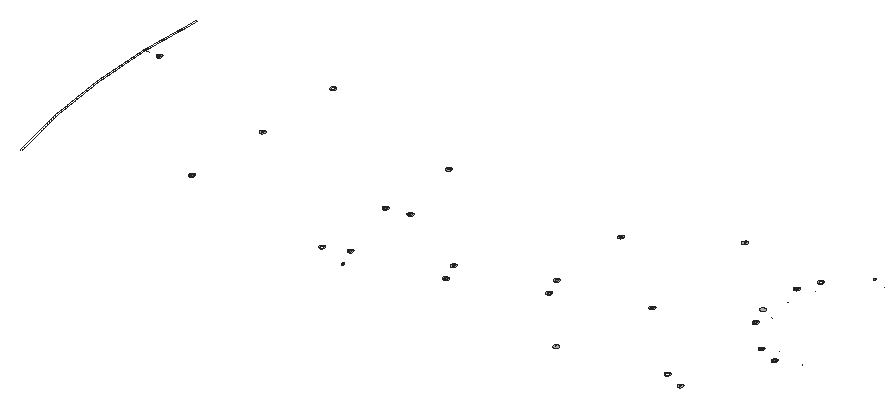
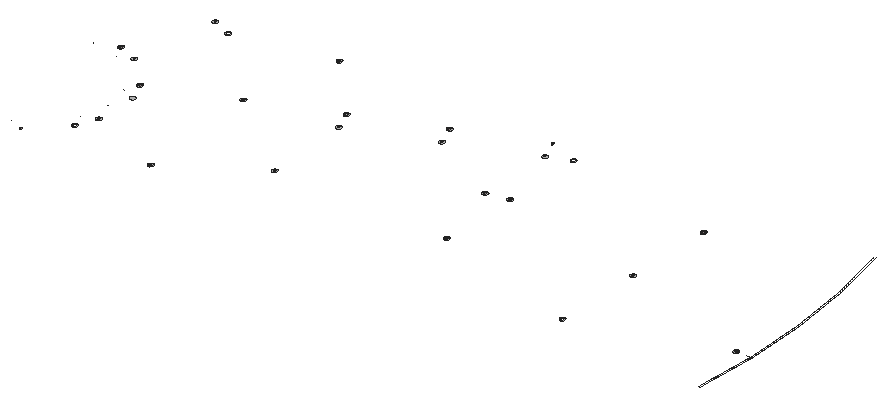
# SketchUp Ruby script. Lengths in inches.
U = 1.inch
M = Sketchup.active_model
def pt(a) = Geom::Point3d.new(a.map { |v| v * U })
def face(e, loops, mat)
  f = e.add_face(loops[0].map { |a| pt(a) })
  loops[1..].each { |l| e.add_face(l.map { |a| pt(a) }).erase! }
  f.material = f.back_material = mat if mat
  f
end
# faces: each face lists its corners as indices into pts; further lists are holes
def faces(e, pts, list, mat = nil) = list.each { |f| face(e, (f[0].is_a?(Array) ? f : [f]).map { |l| l.map { |i| pts[i] } }, mat) }
# xy, xz, yz: faces in a plane at the given z, y or x. An outline is a flat list of corners, or four numbers for a rectangle; further outlines are holes
def ring(l) = l.size == 4 ? [[l[0], l[1]], [l[2], l[1]], [l[2], l[3]], [l[0], l[3]]] : l.each_slice(2).to_a
def flat(e, list, mat, &to3) = list.each { |f| face(e, (f[0].is_a?(Array) ? f : [f]).map { |l| ring(l).map { |u, v| to3.(u, v) } }, mat) }
def xy(e, z, list, mat = nil) = flat(e, list, mat) { |x, y| [x, y, z] }
def xz(e, y, list, mat = nil) = flat(e, list, mat) { |x, z| [x, y, z] }
def yz(e, x, list, mat = nil) = flat(e, list, mat) { |y, z| [x, y, z] }
def lines(e, pts, list) = list.each { |a, b| e.add_line(pt(pts[a]), pt(pts[b])) }
# prism: a flat outline (further loops are holes) pulled along v
def prism(e, loops, v, mat = nil)
  f = face(e, loops, mat); d = Geom::Vector3d.new(v.map { |x| x * U })
  f.pushpull(f.normal.samedirection?(d) ? d.length : -d.length)
end
def box(e, o, s, mat = nil) = prism(e, [[o, [o[0] + s[0], o[1], o[2]], [o[0] + s[0], o[1] + s[1], o[2]], [o[0], o[1] + s[1], o[2]]]], [0, 0, s[2]], mat)
def at(x, y, z, deg = 0) = Geom::Transformation.translation(pt([x, y, z])) * Geom::Transformation.rotation(ORIGIN, Z_AXIS, deg.degrees)
def axes(o, x, y, z) = Geom::Transformation.new([*x, 0, *y, 0, *z, 0, *pt(o).to_a, 1])
def part(name) = M.definitions.add(name)
# library, detail: a bought-in or finely detailed component or shape, given as its bounding box
def library(name, o, s) = part(name).tap { |d| box(d.entities, o, s) }
def detail(e, o, s) = box(e.add_group.entities, o, s)
def put(e, d, t, mat = nil) = e.add_instance(d, t).tap { |i| i.material = mat if mat }
def group(e, t, mat = nil) = e.add_group.tap { |g| g.transformation = t; g.material = mat if mat }.entities
root = M.entities
M.materials.add("[Asphalt_Stamped_Brick]").color = [149, 133, 134]
M.materials.add("[Metal_Steel_Textured_White]").color = [191, 191, 191]
xy(root,3.625,[[147.823,157.497,147.818,157.498,147.8125,157.5,147.809,157.503,147.805,157.507,147.803,157.512,147.803,157.522,147.805,157.527,147.809,157.531,147.8125,157.535,147.818,157.537,147.828,157.537,147.833,157.535,147.837,157.531,147.84,157.527,147.842,157.522,147.843,157.517,147.842,157.512,147.84,157.507,147.837,157.503,147.833,157.5,147.828,157.498],[135.246,157.754,135.241,157.755,135.236,157.757,135.232,157.76,135.229,157.764,135.227,157.769,135.226,157.774,135.227,157.779,135.229,157.784,135.232,157.788,135.236,157.791,135.241,157.793,135.246,157.794,135.252,157.793,135.256,157.791,135.261,157.788,135.264,157.784,135.266,157.779,135.266,157.769,135.264,157.764,135.261,157.76,135.256,157.757,135.252,157.755],[138.456,158.219,138.451,158.22,138.446,158.222,138.442,158.225,138.438,158.229,138.436,158.234,138.436,158.244,138.438,158.249,138.442,158.253,138.446,158.256,138.451,158.258,138.456,158.259,138.461,158.258,138.466,158.256,138.47,158.253,138.473,158.249,138.475,158.244,138.476,158.239,138.475,158.234,138.473,158.229,138.47,158.225,138.466,158.222,138.461,158.22],[128.792,158.391,128.787,158.392,128.782,158.394,128.778,158.397,128.775,158.401,128.773,158.406,128.772,158.411,128.773,158.416,128.775,158.421,128.778,158.425,128.782,158.429,128.787,158.431,128.798,158.431,128.802,158.429,128.807,158.425,128.81,158.421,128.812,158.416,128.8125,158.411,128.812,158.406,128.81,158.401,128.807,158.397,128.802,158.394,128.798,158.392],[138.145,158.957,138.14,158.959,138.136,158.963,138.133,158.967,138.131,158.971,138.13,158.977,138.131,158.982,138.133,158.987,138.136,158.991,138.14,158.994,138.145,158.996,138.15,158.997,138.155,158.996,138.16,158.994,138.164,158.991,138.168,158.987,138.17,158.977,138.169,158.971,138.168,158.967,138.16,158.959,138.155,158.957],
  [141.054,160.159,141.049,160.16,141.044,160.162,141.04,160.165,141.037,160.169,141.035,160.174,141.034,160.179,141.035,160.185,141.037,160.189,141.04,160.194,141.044,160.197,141.049,160.199,141.059,160.199,141.064,160.197,141.068,160.194,141.071,160.189,141.073,160.185,141.074,160.179,141.073,160.174,141.071,160.169,141.068,160.165,141.064,160.162,141.059,160.16],[134.448,160.39,134.443,160.391,134.438,160.393,134.434,160.396,134.431,160.4,134.429,160.405,134.428,160.41,134.429,160.415,134.431,160.42,134.434,160.424,134.438,160.428,134.443,160.43,134.453,160.43,134.458,160.428,134.462,160.424,134.465,160.42,134.467,160.415,134.468,160.41,134.467,160.405,134.465,160.4,134.462,160.396,134.458,160.393,134.453,160.391],[149.025,160.401,149.02,160.402,149.015,160.404,149.011,160.407,149.008,160.411,149.006,160.416,149.005,160.421,149.006,160.426,149.008,160.431,149.011,160.435,149.015,160.438,149.02,160.44,149.025,160.441,149.031,160.44,149.035,160.438,149.04,160.435,149.043,160.431,149.045,160.426,149.045,160.416,149.043,160.411,149.04,160.407,149.035,160.404,149.031,160.402],[135.241,160.556,135.236,160.558,135.232,160.562,135.229,160.566,135.227,160.57,135.226,160.576,135.227,160.581,135.229,160.586,135.232,160.59,135.236,160.593,135.241,160.595,135.246,160.596,135.252,160.595,135.256,160.593,135.261,160.59,135.264,160.586,135.266,160.581,135.266,160.57,135.264,160.566,135.261,160.562,135.256,160.558,135.252,160.556],[144.258,160.625,144.253,160.627,144.249,160.63,144.246,160.635,144.244,160.639,144.243,160.645,144.244,160.65,144.246,160.655,144.249,160.659,144.253,160.662,144.258,160.664,144.263,160.665,144.269,160.664,144.273,160.662,144.277,160.659,144.281,160.655,144.283,160.65,144.283,160.639,144.281,160.635,144.277,160.63,144.273,160.627,144.269,160.625],
  [148.283,160.707,148.278,160.709,148.274,160.713,148.271,160.717,148.269,160.721,148.268,160.727,148.269,160.732,148.271,160.737,148.274,160.741,148.278,160.744,148.283,160.746,148.288,160.747,148.293,160.746,148.298,160.744,148.302,160.741,148.305,160.737,148.307,160.732,148.308,160.727,148.307,160.721,148.305,160.717,148.302,160.713,148.298,160.709,148.293,160.707],[128.792,161.702,128.787,161.703,128.782,161.705,128.778,161.708,128.775,161.712,128.773,161.717,128.772,161.722,128.773,161.727,128.775,161.732,128.778,161.736,128.782,161.739,128.787,161.741,128.792,161.742,128.798,161.741,128.802,161.739,128.807,161.736,128.81,161.732,128.812,161.727,128.8125,161.722,128.812,161.717,128.81,161.712,128.807,161.708,128.802,161.705,128.798,161.703],[147.167,161.827,147.162,161.828,147.157,161.83,147.153,161.833,147.15,161.837,147.148,161.842,147.147,161.847,147.148,161.852,147.15,161.857,147.153,161.861,147.157,161.865,147.162,161.867,147.172,161.867,147.177,161.865,147.181,161.861,147.184,161.857,147.186,161.852,147.187,161.847,147.186,161.842,147.184,161.837,147.181,161.833,147.177,161.83,147.172,161.828],[146.862,164.15,146.856,164.151,146.852,164.153,146.847,164.156,146.844,164.16,146.842,164.165,146.842,164.175,146.844,164.18,146.847,164.184,146.852,164.187,146.856,164.189,146.862,164.19,146.867,164.189,146.872,164.187,146.876,164.184,146.879,164.18,146.881,164.175,146.882,164.17,146.881,164.165,146.879,164.16,146.876,164.156,146.872,164.153,146.867,164.151],[143.953,165.353,143.948,165.355,143.944,165.359,143.941,165.363,143.939,165.367,143.938,165.373,143.939,165.378,143.941,165.383,143.944,165.387,143.948,165.39,143.953,165.392,143.958,165.393,143.963,165.392,143.968,165.39,143.972,165.387,143.975,165.383,143.977,165.378,143.978,165.373,143.977,165.367,143.975,165.363,143.972,165.359,143.968,165.355,143.963,165.353],
  [148.288,166.008,148.283,166.009,148.278,166.011,148.274,166.014,148.271,166.018,148.269,166.023,148.268,166.028,148.269,166.033,148.271,166.038,148.274,166.042,148.278,166.045,148.283,166.047,148.288,166.048,148.293,166.047,148.298,166.045,148.302,166.042,148.305,166.038,148.307,166.033,148.308,166.028,148.307,166.023,148.305,166.018,148.302,166.014,148.298,166.011,148.293,166.009]],"[Asphalt_Stamped_Brick]")
xy(root,3.625,[[[143.513,156.984,143.49,156.987,143.469,156.996,143.451,157.01,143.436,157.029,143.428,157.05,143.425,157.073,143.428,157.096,143.436,157.117,143.451,157.136,143.469,157.15,143.49,157.159,143.513,157.162,143.536,157.159,143.558,157.15,143.576,157.136,143.59,157.117,143.599,157.096,143.602,157.073,143.599,157.05,143.59,157.029,143.576,157.01,143.558,156.996,143.536,156.987],[143.513,156.985,143.536,156.988,143.557,156.997,143.576,157.011,143.59,157.029,143.598,157.05,143.601,157.073,143.598,157.096,143.59,157.117,143.576,157.135,143.557,157.149,143.536,157.158,143.513,157.161,143.491,157.158,143.469,157.149,143.451,157.135,143.437,157.117,143.428,157.096,143.425,157.073,143.428,157.05,143.437,157.029,143.451,157.011,143.469,156.997,143.491,156.988]],[[143.513,156.985,143.491,156.988,143.469,156.997,143.451,157.011,143.437,157.029,143.428,157.05,143.425,157.073,143.428,157.096,143.437,157.117,143.451,157.135,143.469,157.149,143.491,157.158,143.513,157.161,143.536,157.158,143.557,157.149,143.576,157.135,143.59,157.117,143.598,157.096,143.601,157.073,143.598,157.05,143.59,157.029,143.576,157.011,143.557,156.997,143.536,156.988],[143.513,157.036,143.523,157.038,143.532,157.041,143.539,157.047,143.545,157.055,143.549,157.063,143.55,157.073,143.549,157.082,143.545,157.091,143.539,157.099,143.532,157.105,143.523,157.108,143.513,157.11,143.504,157.108,143.495,157.105,143.488,157.099,143.482,157.091,143.478,157.082,143.477,157.073,143.478,157.063,143.482,157.055,143.488,157.047,143.495,157.041,143.504,157.038]],[[135.552,157,135.543,157.001,135.534,157.004,135.526,157.01,135.52,157.018,135.517,157.027,135.515,157.036,135.517,157.046,135.52,157.054,135.526,157.062,135.534,157.068,135.543,157.072,135.552,157.073,135.561,157.072,135.57,157.068,135.578,157.062,135.584,157.054,135.587,157.046,135.589,157.036,135.587,157.027,135.584,157.018,135.578,157.01,135.57,157.004,135.561,157.001],[135.552,157.016,135.557,157.017,135.562,157.019,135.566,157.022,135.569,157.026,135.571,157.031,135.572,157.036,135.571,157.041,135.569,157.046,135.566,157.05,135.562,157.053,135.557,157.055,135.552,157.056,135.547,157.055,135.542,157.053,135.538,157.05,135.535,157.046,135.533,157.041,135.532,157.036,135.533,157.031,135.535,157.026,135.538,157.022,135.542,157.019,135.547,157.017]],[135.552,157.016,135.547,157.017,135.542,157.019,135.538,157.022,135.535,157.026,135.533,157.031,135.532,157.036,135.533,157.041,135.535,157.046,135.538,157.05,135.542,157.053,135.547,157.055,135.552,157.056,135.557,157.055,135.562,157.053,135.566,157.05,135.569,157.046,135.571,157.041,135.572,157.036,135.571,157.031,135.569,157.026,135.566,157.022,135.562,157.019,135.557,157.017],[143.513,157.053,143.508,157.054,143.503,157.056,143.499,157.059,143.496,157.063,143.494,157.068,143.493,157.073,143.494,157.078,143.496,157.083,143.499,157.087,143.503,157.09,143.508,157.092,143.513,157.093,143.519,157.092,143.523,157.09,143.528,157.087,143.531,157.083,143.533,157.078,143.533,157.068,143.531,157.063,143.528,157.059,143.523,157.056,143.519,157.054],
  [[134.448,157.354,134.425,157.357,134.404,157.366,134.385,157.38,134.371,157.399,134.362,157.42,134.359,157.443,134.362,157.466,134.371,157.488,134.385,157.506,134.404,157.52,134.425,157.529,134.448,157.532,134.471,157.529,134.492,157.52,134.511,157.506,134.525,157.488,134.534,157.466,134.537,157.443,134.534,157.42,134.525,157.399,134.511,157.38,134.492,157.366,134.471,157.357],[134.448,157.355,134.471,157.358,134.492,157.367,134.51,157.381,134.524,157.399,134.533,157.42,134.536,157.443,134.533,157.466,134.524,157.487,134.51,157.505,134.492,157.519,134.471,157.528,134.448,157.531,134.425,157.528,134.404,157.519,134.386,157.505,134.372,157.487,134.363,157.466,134.36,157.443,134.363,157.42,134.372,157.399,134.386,157.381,134.404,157.367,134.425,157.358]],[[147.823,157.429,147.8,157.432,147.779,157.441,147.76,157.455,147.747,157.473,147.738,157.495,147.735,157.517,147.738,157.54,147.747,157.561,147.76,157.579,147.779,157.593,147.8,157.602,147.823,157.605,147.845,157.602,147.867,157.593,147.885,157.579,147.899,157.561,147.908,157.54,147.911,157.517,147.908,157.495,147.899,157.473,147.885,157.455,147.867,157.441,147.845,157.432],[147.823,157.481,147.832,157.482,147.841,157.486,147.849,157.491,147.854,157.499,147.858,157.508,147.859,157.517,147.858,157.527,147.854,157.536,147.849,157.543,147.841,157.549,147.832,157.553,147.823,157.554,147.813,157.553,147.804,157.549,147.797,157.543,147.791,157.536,147.787,157.527,147.786,157.517,147.787,157.508,147.791,157.499,147.797,157.491,147.804,157.486,147.813,157.482]],[[147.823,157.481,147.813,157.482,147.804,157.486,147.797,157.491,147.791,157.499,147.787,157.508,147.786,157.517,147.787,157.527,147.791,157.536,147.797,157.543,147.804,157.549,147.813,157.553,147.823,157.554,147.832,157.553,147.841,157.549,147.849,157.543,147.854,157.536,147.858,157.527,147.859,157.517,147.858,157.508,147.854,157.499,147.849,157.491,147.841,157.486,147.832,157.482],[147.823,157.497,147.828,157.498,147.833,157.5,147.837,157.503,147.84,157.507,147.842,157.512,147.843,157.517,147.842,157.522,147.84,157.527,147.837,157.531,147.833,157.535,147.828,157.537,147.818,157.537,147.8125,157.535,147.809,157.531,147.805,157.527,147.803,157.522,147.803,157.512,147.805,157.507,147.809,157.503,147.8125,157.5,147.818,157.498]],[[135.246,157.686,135.224,157.689,135.202,157.698,135.184,157.712,135.17,157.73,135.161,157.751,135.159,157.774,135.161,157.797,135.17,157.818,135.184,157.836,135.202,157.85,135.224,157.859,135.246,157.862,135.269,157.859,135.29,157.85,135.309,157.836,135.323,157.818,135.331,157.797,135.334,157.774,135.331,157.751,135.323,157.73,135.309,157.712,135.29,157.698,135.269,157.689],[135.246,157.737,135.256,157.738,135.265,157.742,135.272,157.748,135.278,157.756,135.282,157.764,135.283,157.774,135.282,157.783,135.278,157.792,135.272,157.8,135.265,157.806,135.256,157.809,135.246,157.81,135.237,157.809,135.228,157.806,135.221,157.8,135.215,157.792,135.211,157.783,135.21,157.774,135.211,157.764,135.215,157.756,135.221,157.748,135.228,157.742,135.237,157.738]],[[147.085,157.734,147.062,157.737,147.041,157.746,147.022,157.76,147.008,157.778,146.999,157.8,146.996,157.823,146.999,157.846,147.008,157.867,147.022,157.886,147.041,157.9,147.062,157.909,147.085,157.912,147.108,157.909,147.129,157.9,147.148,157.886,147.162,157.867,147.171,157.846,147.174,157.823,147.171,157.8,147.162,157.778,147.148,157.76,147.129,157.746,147.108,157.737],[147.085,157.735,147.108,157.738,147.129,157.747,147.147,157.761,147.161,157.779,147.17,157.8,147.173,157.823,147.17,157.846,147.161,157.867,147.147,157.885,147.129,157.899,147.108,157.908,147.085,157.911,147.062,157.908,147.041,157.899,147.023,157.885,147.009,157.867,147,157.846,146.997,157.823,147,157.8,147.009,157.779,147.023,157.761,147.041,157.747,147.062,157.738]],
  [[135.246,157.737,135.237,157.738,135.228,157.742,135.221,157.748,135.215,157.756,135.211,157.764,135.21,157.774,135.211,157.783,135.215,157.792,135.221,157.8,135.228,157.806,135.237,157.809,135.246,157.81,135.256,157.809,135.265,157.806,135.272,157.8,135.278,157.792,135.282,157.783,135.283,157.774,135.282,157.764,135.278,157.756,135.272,157.748,135.265,157.742,135.256,157.738],[135.246,157.754,135.252,157.755,135.256,157.757,135.261,157.76,135.264,157.764,135.266,157.769,135.266,157.779,135.264,157.784,135.261,157.788,135.256,157.791,135.252,157.793,135.246,157.794,135.241,157.793,135.236,157.791,135.232,157.788,135.229,157.784,135.227,157.779,135.226,157.774,135.227,157.769,135.229,157.764,135.232,157.76,135.236,157.757,135.241,157.755]],[[138.456,158.15,138.433,158.153,138.411,158.162,138.393,158.176,138.379,158.195,138.37,158.216,138.367,158.239,138.37,158.262,138.379,158.283,138.393,158.302,138.411,158.316,138.433,158.325,138.456,158.328,138.479,158.325,138.5,158.316,138.519,158.302,138.533,158.283,138.542,158.262,138.545,158.239,138.542,158.216,138.533,158.195,138.519,158.176,138.5,158.162,138.479,158.153],[138.456,158.151,138.479,158.154,138.5,158.163,138.518,158.177,138.532,158.195,138.541,158.216,138.544,158.239,138.541,158.262,138.532,158.283,138.518,158.301,138.5,158.315,138.479,158.324,138.456,158.327,138.433,158.324,138.412,158.315,138.394,158.301,138.38,158.283,138.371,158.262,138.368,158.239,138.371,158.216,138.38,158.195,138.394,158.177,138.412,158.163,138.433,158.154]],[[138.456,158.151,138.433,158.154,138.412,158.163,138.394,158.177,138.38,158.195,138.371,158.216,138.368,158.239,138.371,158.262,138.38,158.283,138.394,158.301,138.412,158.315,138.433,158.324,138.456,158.327,138.479,158.324,138.5,158.315,138.518,158.301,138.532,158.283,138.541,158.262,138.544,158.239,138.541,158.216,138.532,158.195,138.518,158.177,138.5,158.163,138.479,158.154],[138.456,158.202,138.465,158.204,138.474,158.207,138.482,158.213,138.487,158.221,138.491,158.229,138.492,158.239,138.491,158.248,138.487,158.257,138.482,158.265,138.474,158.271,138.465,158.274,138.456,158.276,138.446,158.274,138.4375,158.271,138.43,158.265,138.424,158.257,138.42,158.248,138.419,158.239,138.42,158.229,138.424,158.221,138.43,158.213,138.4375,158.207,138.446,158.204]],[[138.456,158.202,138.446,158.204,138.4375,158.207,138.43,158.213,138.424,158.221,138.42,158.229,138.419,158.239,138.42,158.248,138.424,158.257,138.43,158.265,138.4375,158.271,138.446,158.274,138.456,158.276,138.465,158.274,138.474,158.271,138.482,158.265,138.487,158.257,138.491,158.248,138.492,158.239,138.491,158.229,138.487,158.221,138.482,158.213,138.474,158.207,138.465,158.204],[138.456,158.219,138.461,158.22,138.466,158.222,138.47,158.225,138.473,158.229,138.475,158.234,138.476,158.239,138.475,158.244,138.473,158.249,138.47,158.253,138.466,158.256,138.461,158.258,138.456,158.259,138.451,158.258,138.446,158.256,138.442,158.253,138.438,158.249,138.436,158.244,138.436,158.234,138.438,158.229,138.442,158.225,138.446,158.222,138.451,158.22]],[[128.792,158.322,128.769,158.325,128.748,158.334,128.73,158.348,128.715,158.367,128.707,158.388,128.704,158.411,128.707,158.434,128.715,158.456,128.73,158.474,128.748,158.488,128.769,158.497,128.792,158.5,128.815,158.497,128.837,158.488,128.855,158.474,128.869,158.456,128.878,158.434,128.881,158.411,128.878,158.388,128.869,158.367,128.855,158.348,128.837,158.334,128.815,158.325],[128.792,158.323,128.815,158.326,128.836,158.335,128.855,158.349,128.869,158.367,128.877,158.389,128.88,158.411,128.877,158.434,128.869,158.455,128.855,158.473,128.836,158.487,128.815,158.496,128.792,158.499,128.77,158.496,128.748,158.487,128.73,158.473,128.716,158.455,128.707,158.434,128.704,158.411,128.707,158.389,128.716,158.367,128.73,158.349,128.748,158.335,128.77,158.326]],
  [[128.792,158.375,128.783,158.376,128.774,158.38,128.767,158.385,128.761,158.393,128.757,158.402,128.756,158.411,128.757,158.421,128.761,158.43,128.767,158.437,128.774,158.443,128.783,158.447,128.792,158.448,128.802,158.447,128.811,158.443,128.818,158.437,128.824,158.43,128.828,158.421,128.829,158.411,128.828,158.402,128.824,158.393,128.818,158.385,128.811,158.38,128.802,158.376],[128.792,158.391,128.798,158.392,128.802,158.394,128.807,158.397,128.81,158.401,128.812,158.406,128.8125,158.411,128.812,158.416,128.81,158.421,128.807,158.425,128.802,158.429,128.798,158.431,128.787,158.431,128.782,158.429,128.778,158.425,128.775,158.421,128.773,158.416,128.772,158.411,128.773,158.406,128.775,158.401,128.778,158.397,128.782,158.394,128.787,158.392]],[[138.15,158.889,138.127,158.892,138.106,158.9,138.088,158.914,138.074,158.933,138.065,158.954,138.062,158.977,138.065,158.999,138.074,159.021,138.088,159.039,138.106,159.053,138.127,159.062,138.15,159.065,138.173,159.062,138.194,159.053,138.212,159.039,138.226,159.021,138.235,158.999,138.238,158.977,138.235,158.954,138.226,158.933,138.212,158.914,138.194,158.9,138.173,158.892],[138.15,158.94,138.16,158.941,138.169,158.945,138.176,158.951,138.182,158.958,138.186,158.967,138.187,158.977,138.186,158.986,138.182,158.995,138.176,159.002,138.169,159.008,138.16,159.012,138.15,159.013,138.141,159.012,138.132,159.008,138.124,159.002,138.119,158.995,138.115,158.986,138.114,158.977,138.115,158.967,138.119,158.958,138.124,158.951,138.132,158.945,138.141,158.941]],[[138.15,158.94,138.141,158.941,138.132,158.945,138.124,158.951,138.119,158.958,138.115,158.967,138.114,158.977,138.115,158.986,138.119,158.995,138.124,159.002,138.132,159.008,138.141,159.012,138.15,159.013,138.16,159.012,138.169,159.008,138.176,159.002,138.182,158.995,138.186,158.986,138.187,158.977,138.186,158.967,138.182,158.958,138.176,158.951,138.169,158.945,138.16,158.941],[138.145,158.957,138.155,158.957,138.16,158.959,138.168,158.967,138.169,158.971,138.17,158.977,138.168,158.987,138.164,158.991,138.16,158.994,138.155,158.996,138.15,158.997,138.145,158.996,138.14,158.994,138.136,158.991,138.133,158.987,138.131,158.982,138.13,158.977,138.131,158.971,138.133,158.967,138.136,158.963,138.14,158.959]],[[141.36,159.353,141.337,159.356,141.315,159.365,141.297,159.379,141.283,159.397,141.274,159.419,141.271,159.442,141.274,159.465,141.283,159.486,141.297,159.505,141.315,159.519,141.337,159.528,141.36,159.531,141.383,159.528,141.404,159.519,141.422,159.505,141.437,159.486,141.445,159.465,141.448,159.442,141.445,159.419,141.437,159.397,141.422,159.379,141.404,159.365,141.383,159.356],[141.36,159.354,141.382,159.357,141.404,159.366,141.422,159.38,141.436,159.398,141.444,159.419,141.447,159.442,141.444,159.465,141.436,159.486,141.422,159.504,141.404,159.518,141.382,159.527,141.36,159.53,141.337,159.527,141.316,159.518,141.297,159.504,141.283,159.486,141.275,159.465,141.272,159.442,141.275,159.419,141.283,159.398,141.297,159.38,141.316,159.366,141.337,159.357]],[141.354,159.422,141.35,159.424,141.345,159.428,141.342,159.432,141.34,159.437,141.34,159.447,141.342,159.452,141.345,159.456,141.35,159.459,141.354,159.461,141.36,159.462,141.365,159.461,141.37,159.459,141.374,159.456,141.377,159.452,141.379,159.447,141.38,159.442,141.379,159.437,141.377,159.432,141.374,159.428,141.37,159.424,141.365,159.422],
  [[141.054,160.091,141.031,160.094,141.01,160.103,140.992,160.117,140.978,160.135,140.969,160.157,140.966,160.179,140.969,160.202,140.978,160.223,140.992,160.242,141.01,160.256,141.031,160.264,141.054,160.267,141.077,160.264,141.098,160.256,141.116,160.242,141.13,160.223,141.139,160.202,141.142,160.179,141.139,160.157,141.13,160.135,141.116,160.117,141.098,160.103,141.077,160.094],[141.054,160.143,141.063,160.144,141.072,160.148,141.08,160.154,141.086,160.161,141.089,160.17,141.091,160.179,141.089,160.189,141.086,160.198,141.08,160.205,141.072,160.211,141.063,160.215,141.054,160.216,141.045,160.215,141.036,160.211,141.028,160.205,141.022,160.198,141.019,160.189,141.017,160.179,141.019,160.17,141.022,160.161,141.028,160.154,141.036,160.148,141.045,160.144]],[[141.054,160.143,141.045,160.144,141.036,160.148,141.028,160.154,141.022,160.161,141.019,160.17,141.017,160.179,141.019,160.189,141.022,160.198,141.028,160.205,141.036,160.211,141.045,160.215,141.054,160.216,141.063,160.215,141.072,160.211,141.08,160.205,141.086,160.198,141.089,160.189,141.091,160.179,141.089,160.17,141.086,160.161,141.08,160.154,141.072,160.148,141.063,160.144],[141.054,160.159,141.059,160.16,141.064,160.162,141.068,160.165,141.071,160.169,141.073,160.174,141.074,160.179,141.073,160.185,141.071,160.189,141.068,160.194,141.064,160.197,141.059,160.199,141.049,160.199,141.044,160.197,141.04,160.194,141.037,160.189,141.035,160.185,141.034,160.179,141.035,160.174,141.037,160.169,141.04,160.165,141.044,160.162,141.049,160.16]],[[134.448,160.321,134.425,160.324,134.404,160.333,134.385,160.347,134.371,160.366,134.362,160.387,134.359,160.41,134.362,160.433,134.371,160.455,134.385,160.473,134.404,160.487,134.425,160.496,134.448,160.499,134.471,160.496,134.492,160.487,134.511,160.473,134.525,160.455,134.534,160.433,134.537,160.41,134.534,160.387,134.525,160.366,134.511,160.347,134.492,160.333,134.471,160.324],[134.448,160.322,134.471,160.325,134.492,160.334,134.51,160.348,134.524,160.366,134.533,160.388,134.536,160.41,134.533,160.433,134.524,160.454,134.51,160.472,134.492,160.486,134.471,160.495,134.448,160.498,134.425,160.495,134.404,160.486,134.386,160.472,134.372,160.454,134.363,160.433,134.36,160.41,134.363,160.388,134.372,160.366,134.386,160.348,134.404,160.334,134.425,160.325]],[[149.025,160.332,149.002,160.335,148.981,160.344,148.963,160.358,148.948,160.377,148.94,160.398,148.937,160.421,148.94,160.444,148.948,160.466,148.963,160.484,148.981,160.498,149.002,160.507,149.025,160.51,149.048,160.507,149.07,160.498,149.088,160.484,149.102,160.466,149.111,160.444,149.114,160.421,149.111,160.398,149.102,160.377,149.088,160.358,149.07,160.344,149.048,160.335],[149.025,160.333,149.048,160.336,149.069,160.345,149.088,160.359,149.102,160.377,149.11,160.398,149.113,160.421,149.11,160.444,149.102,160.465,149.088,160.483,149.069,160.497,149.048,160.506,149.025,160.509,149.003,160.506,148.981,160.497,148.963,160.483,148.949,160.465,148.941,160.444,148.9375,160.421,148.941,160.398,148.949,160.377,148.963,160.359,148.981,160.345,149.003,160.336]],[[134.448,160.374,134.439,160.375,134.43,160.379,134.422,160.384,134.416,160.392,134.413,160.401,134.411,160.41,134.413,160.42,134.416,160.429,134.422,160.436,134.43,160.442,134.439,160.446,134.448,160.447,134.457,160.446,134.466,160.442,134.474,160.436,134.48,160.429,134.483,160.42,134.485,160.41,134.483,160.401,134.48,160.392,134.474,160.384,134.466,160.379,134.457,160.375],[134.448,160.39,134.453,160.391,134.458,160.393,134.462,160.396,134.465,160.4,134.467,160.405,134.468,160.41,134.467,160.415,134.465,160.42,134.462,160.424,134.458,160.428,134.453,160.43,134.443,160.43,134.438,160.428,134.434,160.424,134.431,160.42,134.429,160.415,134.428,160.41,134.429,160.405,134.431,160.4,134.434,160.396,134.438,160.393,134.443,160.391]],
  [[149.025,160.385,149.016,160.386,149.007,160.389,149,160.395,148.994,160.403,148.99,160.412,148.989,160.421,148.99,160.431,148.994,160.439,149,160.447,149.007,160.453,149.016,160.456,149.025,160.458,149.035,160.456,149.044,160.453,149.051,160.447,149.057,160.439,149.061,160.431,149.062,160.421,149.061,160.412,149.057,160.403,149.051,160.395,149.044,160.389,149.035,160.386],[149.025,160.401,149.031,160.402,149.035,160.404,149.04,160.407,149.043,160.411,149.045,160.416,149.045,160.426,149.043,160.431,149.04,160.435,149.035,160.438,149.031,160.44,149.025,160.441,149.02,160.44,149.015,160.438,149.011,160.435,149.008,160.431,149.006,160.426,149.005,160.421,149.006,160.416,149.008,160.411,149.011,160.407,149.015,160.404,149.02,160.402]],[[135.246,160.487,135.223,160.49,135.202,160.499,135.184,160.513,135.169,160.531,135.161,160.553,135.158,160.576,135.161,160.599,135.169,160.62,135.184,160.638,135.202,160.653,135.223,160.661,135.246,160.665,135.269,160.661,135.291,160.653,135.309,160.638,135.323,160.62,135.332,160.599,135.335,160.576,135.332,160.553,135.323,160.531,135.309,160.513,135.291,160.499,135.269,160.49],[135.246,160.488,135.269,160.491,135.29,160.499,135.309,160.513,135.323,160.532,135.331,160.553,135.334,160.576,135.331,160.598,135.323,160.62,135.309,160.638,135.29,160.652,135.269,160.661,135.246,160.664,135.224,160.661,135.202,160.652,135.184,160.638,135.17,160.62,135.161,160.598,135.159,160.576,135.161,160.553,135.17,160.532,135.184,160.513,135.202,160.499,135.224,160.491]],[[135.246,160.488,135.224,160.491,135.202,160.499,135.184,160.513,135.17,160.532,135.161,160.553,135.159,160.576,135.161,160.598,135.17,160.62,135.184,160.638,135.202,160.652,135.224,160.661,135.246,160.664,135.269,160.661,135.29,160.652,135.309,160.638,135.323,160.62,135.331,160.598,135.334,160.576,135.331,160.553,135.323,160.532,135.309,160.513,135.29,160.499,135.269,160.491],[135.246,160.539,135.256,160.54,135.265,160.544,135.272,160.55,135.278,160.557,135.282,160.566,135.283,160.576,135.282,160.585,135.278,160.594,135.272,160.602,135.265,160.607,135.256,160.611,135.246,160.612,135.237,160.611,135.228,160.607,135.221,160.602,135.215,160.594,135.211,160.585,135.21,160.576,135.211,160.566,135.215,160.557,135.221,160.55,135.228,160.544,135.237,160.54]],[[135.246,160.539,135.237,160.54,135.228,160.544,135.221,160.55,135.215,160.557,135.211,160.566,135.21,160.576,135.211,160.585,135.215,160.594,135.221,160.602,135.228,160.607,135.237,160.611,135.246,160.612,135.256,160.611,135.265,160.607,135.272,160.602,135.278,160.594,135.282,160.585,135.283,160.576,135.282,160.566,135.278,160.557,135.272,160.55,135.265,160.544,135.256,160.54],[135.241,160.556,135.252,160.556,135.256,160.558,135.261,160.562,135.264,160.566,135.266,160.57,135.266,160.581,135.264,160.586,135.261,160.59,135.256,160.593,135.252,160.595,135.246,160.596,135.241,160.595,135.236,160.593,135.232,160.59,135.229,160.586,135.227,160.581,135.226,160.576,135.227,160.57,135.229,160.566,135.232,160.562,135.236,160.558]],[[144.263,160.556,144.24,160.559,144.219,160.568,144.2,160.582,144.186,160.6,144.177,160.622,144.174,160.645,144.177,160.668,144.186,160.689,144.2,160.707,144.219,160.722,144.24,160.73,144.263,160.733,144.286,160.73,144.308,160.722,144.326,160.707,144.34,160.689,144.349,160.668,144.352,160.645,144.349,160.622,144.34,160.6,144.326,160.582,144.308,160.568,144.286,160.559],[144.263,160.557,144.286,160.56,144.307,160.568,144.326,160.582,144.339,160.601,144.348,160.622,144.351,160.645,144.348,160.667,144.339,160.689,144.326,160.707,144.307,160.721,144.286,160.729,144.263,160.732,144.241,160.729,144.219,160.721,144.201,160.707,144.187,160.689,144.178,160.667,144.175,160.645,144.178,160.622,144.187,160.601,144.201,160.582,144.219,160.568,144.241,160.56]],
  [[144.263,160.608,144.254,160.609,144.245,160.613,144.237,160.619,144.232,160.626,144.228,160.635,144.227,160.645,144.228,160.654,144.232,160.663,144.237,160.67,144.245,160.676,144.254,160.68,144.263,160.681,144.273,160.68,144.282,160.676,144.289,160.67,144.295,160.663,144.299,160.654,144.3,160.645,144.299,160.635,144.295,160.626,144.289,160.619,144.282,160.613,144.273,160.609],[144.258,160.625,144.269,160.625,144.273,160.627,144.277,160.63,144.281,160.635,144.283,160.639,144.283,160.65,144.281,160.655,144.277,160.659,144.273,160.662,144.269,160.664,144.263,160.665,144.258,160.664,144.253,160.662,144.249,160.659,144.246,160.655,144.244,160.65,144.243,160.645,144.244,160.639,144.246,160.635,144.249,160.63,144.253,160.627]],[[148.288,160.638,148.265,160.641,148.243,160.65,148.225,160.664,148.211,160.682,148.202,160.704,148.199,160.727,148.202,160.75,148.211,160.771,148.225,160.79,148.243,160.804,148.265,160.8125,148.288,160.816,148.311,160.8125,148.332,160.804,148.351,160.79,148.365,160.771,148.374,160.75,148.377,160.727,148.374,160.704,148.365,160.682,148.351,160.664,148.332,160.65,148.311,160.641],[148.288,160.639,148.311,160.642,148.332,160.651,148.35,160.664,148.364,160.683,148.373,160.704,148.376,160.727,148.373,160.749,148.364,160.771,148.35,160.789,148.332,160.803,148.311,160.812,148.288,160.815,148.265,160.812,148.244,160.803,148.226,160.789,148.212,160.771,148.203,160.749,148.2,160.727,148.203,160.704,148.212,160.683,148.226,160.664,148.244,160.651,148.265,160.642]],[[148.288,160.639,148.265,160.642,148.244,160.651,148.226,160.664,148.212,160.683,148.203,160.704,148.2,160.727,148.203,160.749,148.212,160.771,148.226,160.789,148.244,160.803,148.265,160.812,148.288,160.815,148.311,160.812,148.332,160.803,148.35,160.789,148.364,160.771,148.373,160.749,148.376,160.727,148.373,160.704,148.364,160.683,148.35,160.664,148.332,160.651,148.311,160.642],[148.288,160.69,148.297,160.691,148.306,160.695,148.314,160.701,148.319,160.708,148.323,160.717,148.324,160.727,148.323,160.736,148.319,160.745,148.314,160.753,148.306,160.758,148.297,160.762,148.288,160.763,148.278,160.762,148.27,160.758,148.262,160.753,148.256,160.745,148.252,160.736,148.251,160.727,148.252,160.717,148.256,160.708,148.262,160.701,148.27,160.695,148.278,160.691]],[[148.288,160.69,148.278,160.691,148.27,160.695,148.262,160.701,148.256,160.708,148.252,160.717,148.251,160.727,148.252,160.736,148.256,160.745,148.262,160.753,148.27,160.758,148.278,160.762,148.288,160.763,148.297,160.762,148.306,160.758,148.314,160.753,148.319,160.745,148.323,160.736,148.324,160.727,148.323,160.717,148.319,160.708,148.314,160.701,148.306,160.695,148.297,160.691],[148.283,160.707,148.293,160.707,148.298,160.709,148.302,160.713,148.305,160.717,148.307,160.721,148.308,160.727,148.307,160.732,148.305,160.737,148.302,160.741,148.298,160.744,148.293,160.746,148.288,160.747,148.283,160.746,148.278,160.744,148.274,160.741,148.271,160.737,148.269,160.732,148.268,160.727,148.269,160.721,148.271,160.717,148.274,160.713,148.278,160.709]],[[128.792,161.634,128.77,161.637,128.748,161.646,128.73,161.66,128.716,161.678,128.707,161.699,128.704,161.722,128.707,161.745,128.716,161.766,128.73,161.784,128.748,161.798,128.77,161.807,128.792,161.81,128.815,161.807,128.836,161.798,128.855,161.784,128.869,161.766,128.877,161.745,128.88,161.722,128.877,161.699,128.869,161.678,128.855,161.66,128.836,161.646,128.815,161.637],[128.792,161.685,128.802,161.687,128.811,161.69,128.818,161.696,128.824,161.704,128.828,161.713,128.829,161.722,128.828,161.732,128.824,161.74,128.818,161.748,128.811,161.754,128.802,161.757,128.792,161.759,128.783,161.757,128.774,161.754,128.767,161.748,128.761,161.74,128.757,161.732,128.756,161.722,128.757,161.713,128.761,161.704,128.767,161.696,128.774,161.69,128.783,161.687]],
  [[128.792,161.685,128.783,161.687,128.774,161.69,128.767,161.696,128.761,161.704,128.757,161.713,128.756,161.722,128.757,161.732,128.761,161.74,128.767,161.748,128.774,161.754,128.783,161.757,128.792,161.759,128.802,161.757,128.811,161.754,128.818,161.748,128.824,161.74,128.828,161.732,128.829,161.722,128.828,161.713,128.824,161.704,128.818,161.696,128.811,161.69,128.802,161.687],[128.792,161.702,128.798,161.703,128.802,161.705,128.807,161.708,128.81,161.712,128.812,161.717,128.8125,161.722,128.812,161.727,128.81,161.732,128.807,161.736,128.802,161.739,128.798,161.741,128.792,161.742,128.787,161.741,128.782,161.739,128.778,161.736,128.775,161.732,128.773,161.727,128.772,161.722,128.773,161.717,128.775,161.712,128.778,161.708,128.782,161.705,128.787,161.703]],[[147.167,161.758,147.144,161.761,147.123,161.77,147.104,161.784,147.09,161.803,147.081,161.824,147.078,161.847,147.081,161.87,147.09,161.892,147.104,161.91,147.123,161.924,147.144,161.933,147.167,161.936,147.19,161.933,147.212,161.924,147.23,161.91,147.244,161.892,147.253,161.87,147.256,161.847,147.253,161.824,147.244,161.803,147.23,161.784,147.212,161.77,147.19,161.761],[147.167,161.759,147.19,161.762,147.211,161.771,147.229,161.785,147.243,161.803,147.252,161.825,147.255,161.847,147.252,161.87,147.243,161.891,147.229,161.91,147.211,161.923,147.19,161.932,147.167,161.935,147.144,161.932,147.123,161.923,147.105,161.91,147.091,161.891,147.082,161.87,147.079,161.847,147.082,161.825,147.091,161.803,147.105,161.785,147.123,161.771,147.144,161.762]],[[147.167,161.759,147.144,161.762,147.123,161.771,147.105,161.785,147.091,161.803,147.082,161.825,147.079,161.847,147.082,161.87,147.091,161.891,147.105,161.91,147.123,161.923,147.144,161.932,147.167,161.935,147.19,161.932,147.211,161.923,147.229,161.91,147.243,161.891,147.252,161.87,147.255,161.847,147.252,161.825,147.243,161.803,147.229,161.785,147.211,161.771,147.19,161.762],[147.167,161.811,147.177,161.812,147.185,161.816,147.193,161.821,147.199,161.829,147.202,161.838,147.204,161.847,147.202,161.857,147.199,161.866,147.193,161.873,147.185,161.879,147.177,161.883,147.167,161.884,147.158,161.883,147.149,161.879,147.141,161.873,147.135,161.866,147.132,161.857,147.131,161.847,147.132,161.838,147.135,161.829,147.141,161.821,147.149,161.816,147.158,161.812]],[[147.167,161.811,147.158,161.812,147.149,161.816,147.141,161.821,147.135,161.829,147.132,161.838,147.131,161.847,147.132,161.857,147.135,161.866,147.141,161.873,147.149,161.879,147.158,161.883,147.167,161.884,147.177,161.883,147.185,161.879,147.193,161.873,147.199,161.866,147.202,161.857,147.204,161.847,147.202,161.838,147.199,161.829,147.193,161.821,147.185,161.816,147.177,161.812],[147.167,161.827,147.172,161.828,147.177,161.83,147.181,161.833,147.184,161.837,147.186,161.842,147.187,161.847,147.186,161.852,147.184,161.857,147.181,161.861,147.177,161.865,147.172,161.867,147.162,161.867,147.157,161.865,147.153,161.861,147.15,161.857,147.148,161.852,147.147,161.847,147.148,161.842,147.15,161.837,147.153,161.833,147.157,161.83,147.162,161.828]],[[146.862,162.497,146.839,162.5,146.818,162.509,146.799,162.523,146.785,162.541,146.777,162.562,146.774,162.585,146.777,162.608,146.785,162.629,146.799,162.647,146.818,162.661,146.839,162.67,146.862,162.673,146.884,162.67,146.906,162.661,146.924,162.647,146.938,162.629,146.947,162.608,146.95,162.585,146.947,162.562,146.938,162.541,146.924,162.523,146.906,162.509,146.884,162.5],[146.862,162.548,146.871,162.55,146.88,162.553,146.887,162.559,146.893,162.567,146.897,162.576,146.898,162.585,146.897,162.594,146.893,162.603,146.887,162.611,146.88,162.617,146.871,162.62,146.862,162.622,146.852,162.62,146.843,162.617,146.836,162.611,146.83,162.603,146.826,162.594,146.825,162.585,146.826,162.576,146.83,162.567,146.836,162.559,146.843,162.553,146.852,162.55]],
  [123.603,163.289,123.625,163.292,123.647,163.301,123.665,163.315,123.679,163.333,123.6875,163.355,123.69,163.377,123.691,163.377,123.688,163.354,123.68,163.333,123.665,163.315,123.647,163.3,123.626,163.292,123.603,163.289,123.58,163.292,123.558,163.3,123.54,163.315,123.526,163.333,123.517,163.354,123.514,163.377,123.515,163.377,123.518,163.355,123.526,163.333,123.54,163.315,123.559,163.301,123.58,163.292],[134.448,163.289,134.425,163.292,134.404,163.301,134.386,163.315,134.372,163.333,134.363,163.355,134.36,163.377,134.411,163.377,134.413,163.368,134.416,163.359,134.422,163.352,134.43,163.346,134.439,163.342,134.448,163.341,134.457,163.342,134.466,163.346,134.474,163.352,134.48,163.359,134.483,163.368,134.485,163.377,134.536,163.377,134.533,163.355,134.524,163.333,134.51,163.315,134.492,163.301,134.471,163.292],[[140.902,163.289,140.879,163.292,140.858,163.301,140.84,163.315,140.826,163.333,140.817,163.355,140.814,163.377,140.813,163.377,140.816,163.4,140.825,163.422,140.839,163.44,140.858,163.454,140.879,163.463,140.902,163.466,140.925,163.463,140.946,163.454,140.965,163.44,140.979,163.422,140.988,163.4,140.991,163.377,140.99,163.377,140.987,163.355,140.978,163.333,140.964,163.315,140.946,163.301,140.925,163.292],[140.902,163.341,140.911,163.342,140.92,163.346,140.928,163.352,140.934,163.359,140.9375,163.368,140.939,163.377,140.9375,163.387,140.934,163.396,140.928,163.403,140.92,163.409,140.911,163.413,140.902,163.414,140.893,163.413,140.884,163.409,140.876,163.403,140.87,163.396,140.867,163.387,140.865,163.377,140.867,163.368,140.87,163.359,140.876,163.352,140.884,163.346,140.893,163.342]],[123.603,163.341,123.593,163.342,123.584,163.346,123.577,163.352,123.571,163.359,123.567,163.368,123.566,163.377,123.583,163.377,123.583,163.372,123.585,163.367,123.588,163.363,123.593,163.36,123.597,163.358,123.603,163.357,123.608,163.358,123.613,163.36,123.617,163.363,123.62,163.367,123.622,163.372,123.623,163.377,123.639,163.377,123.638,163.368,123.634,163.359,123.628,163.352,123.621,163.346,123.612,163.342],[140.902,163.341,140.893,163.342,140.884,163.346,140.876,163.352,140.87,163.359,140.867,163.368,140.865,163.377,140.882,163.377,140.883,163.372,140.885,163.367,140.888,163.363,140.892,163.36,140.897,163.358,140.902,163.357,140.907,163.358,140.912,163.36,140.916,163.363,140.919,163.367,140.921,163.372,140.922,163.377,140.939,163.377,140.9375,163.368,140.934,163.359,140.928,163.352,140.92,163.346,140.911,163.342],
  [123.603,163.357,123.597,163.358,123.593,163.36,123.588,163.363,123.585,163.367,123.583,163.372,123.583,163.377,123.623,163.377,123.622,163.372,123.62,163.367,123.617,163.363,123.613,163.36,123.608,163.358],[134.448,163.357,134.443,163.358,134.438,163.36,134.434,163.363,134.431,163.367,134.429,163.372,134.428,163.377,134.468,163.377,134.467,163.372,134.465,163.367,134.462,163.363,134.458,163.36,134.453,163.358],[123.515,163.377,123.518,163.4,123.526,163.421,123.54,163.44,123.559,163.454,123.58,163.462,123.603,163.465,123.625,163.462,123.647,163.454,123.665,163.44,123.679,163.421,123.6875,163.4,123.69,163.377,123.639,163.377,123.638,163.387,123.634,163.396,123.628,163.403,123.621,163.409,123.612,163.413,123.603,163.414,123.593,163.413,123.584,163.409,123.577,163.403,123.571,163.396,123.567,163.387,123.566,163.377],[123.583,163.377,123.583,163.383,123.585,163.387,123.588,163.392,123.593,163.395,123.597,163.397,123.608,163.397,123.613,163.395,123.617,163.392,123.62,163.387,123.622,163.383,123.623,163.377],[134.359,163.377,134.362,163.4,134.371,163.422,134.385,163.44,134.404,163.454,134.425,163.463,134.448,163.466,134.471,163.463,134.492,163.454,134.511,163.44,134.525,163.422,134.534,163.4,134.537,163.377,134.536,163.377,134.533,163.4,134.524,163.421,134.51,163.44,134.492,163.454,134.471,163.462,134.448,163.465,134.425,163.462,134.404,163.454,134.386,163.44,134.372,163.421,134.363,163.4,134.36,163.377],
  [134.411,163.377,134.413,163.387,134.416,163.396,134.422,163.403,134.43,163.409,134.439,163.413,134.448,163.414,134.457,163.413,134.466,163.409,134.474,163.403,134.48,163.396,134.483,163.387,134.485,163.377,134.468,163.377,134.467,163.383,134.465,163.387,134.462,163.392,134.458,163.395,134.453,163.397,134.443,163.397,134.438,163.395,134.434,163.392,134.431,163.387,134.429,163.383,134.428,163.377],[134.428,163.377,134.429,163.383,134.431,163.387,134.434,163.392,134.438,163.395,134.443,163.397,134.453,163.397,134.458,163.395,134.462,163.392,134.465,163.387,134.467,163.383,134.468,163.377],[140.814,163.377,140.817,163.4,140.826,163.421,140.84,163.44,140.858,163.454,140.879,163.462,140.902,163.465,140.925,163.462,140.946,163.454,140.964,163.44,140.978,163.421,140.987,163.4,140.99,163.377,140.939,163.377,140.9375,163.387,140.934,163.396,140.928,163.403,140.92,163.409,140.911,163.413,140.902,163.414,140.893,163.413,140.884,163.409,140.876,163.403,140.87,163.396,140.867,163.387,140.865,163.377],[140.865,163.377,140.867,163.387,140.87,163.396,140.876,163.403,140.884,163.409,140.893,163.413,140.902,163.414,140.911,163.413,140.92,163.409,140.928,163.403,140.934,163.396,140.9375,163.387,140.939,163.377,140.922,163.377,140.921,163.383,140.919,163.387,140.916,163.392,140.912,163.395,140.907,163.397,140.897,163.397,140.892,163.395,140.888,163.392,140.885,163.387,140.883,163.383,140.882,163.377],[140.882,163.377,140.883,163.383,140.885,163.387,140.888,163.392,140.892,163.395,140.897,163.397,140.907,163.397,140.912,163.395,140.916,163.392,140.919,163.387,140.921,163.383,140.922,163.377],
  [[146.862,164.081,146.839,164.084,146.817,164.093,146.799,164.107,146.785,164.125,146.776,164.147,146.773,164.17,146.776,164.193,146.785,164.214,146.799,164.233,146.817,164.247,146.839,164.256,146.862,164.259,146.885,164.256,146.906,164.247,146.924,164.233,146.939,164.214,146.947,164.193,146.95,164.17,146.947,164.147,146.939,164.125,146.924,164.107,146.906,164.093,146.885,164.084],[146.862,164.082,146.884,164.085,146.906,164.094,146.924,164.108,146.938,164.126,146.947,164.147,146.95,164.17,146.947,164.193,146.938,164.214,146.924,164.232,146.906,164.246,146.884,164.255,146.862,164.258,146.839,164.255,146.818,164.246,146.799,164.232,146.785,164.214,146.777,164.193,146.774,164.17,146.777,164.147,146.785,164.126,146.799,164.108,146.818,164.094,146.839,164.085]],[[146.862,164.082,146.839,164.085,146.818,164.094,146.799,164.108,146.785,164.126,146.777,164.147,146.774,164.17,146.777,164.193,146.785,164.214,146.799,164.232,146.818,164.246,146.839,164.255,146.862,164.258,146.884,164.255,146.906,164.246,146.924,164.232,146.938,164.214,146.947,164.193,146.95,164.17,146.947,164.147,146.938,164.126,146.924,164.108,146.906,164.094,146.884,164.085],[146.862,164.133,146.871,164.135,146.88,164.138,146.887,164.144,146.893,164.152,146.897,164.16,146.898,164.17,146.897,164.179,146.893,164.188,146.887,164.196,146.88,164.202,146.871,164.205,146.862,164.206,146.852,164.205,146.843,164.202,146.836,164.196,146.83,164.188,146.826,164.179,146.825,164.17,146.826,164.16,146.83,164.152,146.836,164.144,146.843,164.138,146.852,164.135]],[[146.862,164.133,146.852,164.135,146.843,164.138,146.836,164.144,146.83,164.152,146.826,164.16,146.825,164.17,146.826,164.179,146.83,164.188,146.836,164.196,146.843,164.202,146.852,164.205,146.862,164.206,146.871,164.205,146.88,164.202,146.887,164.196,146.893,164.188,146.897,164.179,146.898,164.17,146.897,164.16,146.893,164.152,146.887,164.144,146.88,164.138,146.871,164.135],[146.862,164.15,146.867,164.151,146.872,164.153,146.876,164.156,146.879,164.16,146.881,164.165,146.882,164.17,146.881,164.175,146.879,164.18,146.876,164.184,146.872,164.187,146.867,164.189,146.862,164.19,146.856,164.189,146.852,164.187,146.847,164.184,146.844,164.18,146.842,164.175,146.842,164.165,146.844,164.16,146.847,164.156,146.852,164.153,146.856,164.151]],[[147.167,164.819,147.144,164.822,147.123,164.831,147.104,164.845,147.09,164.863,147.081,164.885,147.078,164.908,147.081,164.931,147.09,164.952,147.104,164.97,147.123,164.984,147.144,164.993,147.167,164.996,147.19,164.993,147.212,164.984,147.23,164.97,147.244,164.952,147.253,164.931,147.256,164.908,147.253,164.885,147.244,164.863,147.23,164.845,147.212,164.831,147.19,164.822],[147.167,164.82,147.19,164.823,147.211,164.831,147.229,164.845,147.243,164.864,147.252,164.885,147.255,164.908,147.252,164.93,147.243,164.951,147.229,164.97,147.211,164.984,147.19,164.992,147.167,164.995,147.144,164.992,147.123,164.984,147.105,164.97,147.091,164.951,147.082,164.93,147.079,164.908,147.082,164.885,147.091,164.864,147.105,164.845,147.123,164.831,147.144,164.823]],[[128.792,164.944,128.769,164.947,128.748,164.956,128.73,164.97,128.715,164.988,128.707,165.01,128.704,165.033,128.707,165.056,128.715,165.077,128.73,165.096,128.748,165.11,128.769,165.119,128.792,165.122,128.815,165.119,128.837,165.11,128.855,165.096,128.869,165.077,128.878,165.056,128.881,165.033,128.878,165.01,128.869,164.988,128.855,164.97,128.837,164.956,128.815,164.947],[128.792,164.945,128.815,164.948,128.836,164.957,128.855,164.971,128.869,164.989,128.877,165.01,128.88,165.033,128.877,165.056,128.869,165.077,128.855,165.095,128.836,165.109,128.815,165.118,128.792,165.121,128.77,165.118,128.748,165.109,128.73,165.095,128.716,165.077,128.707,165.056,128.704,165.033,128.707,165.01,128.716,164.989,128.73,164.971,128.748,164.957,128.77,164.948]],
  [[143.958,165.284,143.935,165.287,143.913,165.296,143.895,165.31,143.881,165.328,143.872,165.35,143.869,165.373,143.872,165.396,143.881,165.417,143.895,165.435,143.913,165.45,143.935,165.459,143.958,165.462,143.981,165.459,144.002,165.45,144.021,165.435,144.035,165.417,144.044,165.396,144.047,165.373,144.044,165.35,144.035,165.328,144.021,165.31,144.002,165.296,143.981,165.287],[143.958,165.285,143.981,165.288,144.002,165.296,144.02,165.31,144.034,165.329,144.043,165.35,144.046,165.373,144.043,165.395,144.034,165.417,144.02,165.435,144.002,165.449,143.981,165.458,143.958,165.461,143.935,165.458,143.914,165.449,143.896,165.435,143.882,165.417,143.873,165.395,143.87,165.373,143.873,165.35,143.882,165.329,143.896,165.31,143.914,165.296,143.935,165.288]],[[143.958,165.285,143.935,165.288,143.914,165.296,143.896,165.31,143.882,165.329,143.873,165.35,143.87,165.373,143.873,165.395,143.882,165.417,143.896,165.435,143.914,165.449,143.935,165.458,143.958,165.461,143.981,165.458,144.002,165.449,144.02,165.435,144.034,165.417,144.043,165.395,144.046,165.373,144.043,165.35,144.034,165.329,144.02,165.31,144.002,165.296,143.981,165.288],[143.958,165.336,143.967,165.337,143.976,165.341,143.984,165.347,143.989,165.354,143.993,165.363,143.994,165.373,143.993,165.382,143.989,165.391,143.984,165.399,143.976,165.404,143.967,165.408,143.958,165.409,143.948,165.408,143.939,165.404,143.932,165.399,143.926,165.391,143.922,165.382,143.921,165.373,143.922,165.363,143.926,165.354,143.932,165.347,143.939,165.341,143.948,165.337]],[[143.958,165.336,143.948,165.337,143.939,165.341,143.932,165.347,143.926,165.354,143.922,165.363,143.921,165.373,143.922,165.382,143.926,165.391,143.932,165.399,143.939,165.404,143.948,165.408,143.958,165.409,143.967,165.408,143.976,165.404,143.984,165.399,143.989,165.391,143.993,165.382,143.994,165.373,143.993,165.363,143.989,165.354,143.984,165.347,143.976,165.341,143.967,165.337],[143.953,165.353,143.963,165.353,143.968,165.355,143.972,165.359,143.975,165.363,143.977,165.367,143.978,165.373,143.977,165.378,143.975,165.383,143.972,165.387,143.968,165.39,143.963,165.392,143.958,165.393,143.953,165.392,143.948,165.39,143.944,165.387,143.941,165.383,143.939,165.378,143.938,165.373,143.939,165.367,143.941,165.363,143.944,165.359,143.948,165.355]],[[148.288,165.992,148.278,165.993,148.27,165.996,148.262,166.002,148.256,166.01,148.252,166.019,148.251,166.028,148.252,166.038,148.256,166.046,148.262,166.054,148.27,166.06,148.278,166.064,148.288,166.065,148.297,166.064,148.306,166.06,148.314,166.054,148.319,166.046,148.323,166.038,148.324,166.028,148.323,166.019,148.319,166.01,148.314,166.002,148.306,165.996,148.297,165.993],[148.288,166.008,148.293,166.009,148.298,166.011,148.302,166.014,148.305,166.018,148.307,166.023,148.308,166.028,148.307,166.033,148.305,166.038,148.302,166.042,148.298,166.045,148.293,166.047,148.288,166.048,148.283,166.047,148.278,166.045,148.274,166.042,148.271,166.038,148.269,166.033,148.268,166.028,148.269,166.023,148.271,166.018,148.274,166.014,148.278,166.011,148.283,166.009]]],"[Metal_Steel_Textured_White]")
p = [[147.17,163.377,3.625],[147.156,163.377,3.625],[123.07,163.377,3.625],[123.004,163.377,3.625],[123.203,163.377,3.625],[148.804,160.931,3.625],
  [148.799,160.919,3.625],[147.371,164.391,3.625],[147.359,164.396,3.625],[149.818,160.729,3.625],[149.818,160.716,3.625],[123.172,165.709,3.625],
  [123.106,165.714,3.625],[123.106,161.04,3.625],[123.411,158.721,3.625],[123.917,156.4375,3.625],[123.172,161.046,3.625],[123.477,158.733,3.625],
  [123.982,156.455,3.625],[147.359,162.359,3.625],[147.371,162.364,3.625],[148.799,165.836,3.625],[148.804,165.824,3.625]]
lines(root,p,[[0,1],[2,3],[4,2],[5,6],[7,8],[9,10],[11,2],[12,3],[3,13],[13,14],[14,15],[16,17],
  [17,18],[2,16],[19,20],[21,22]])
